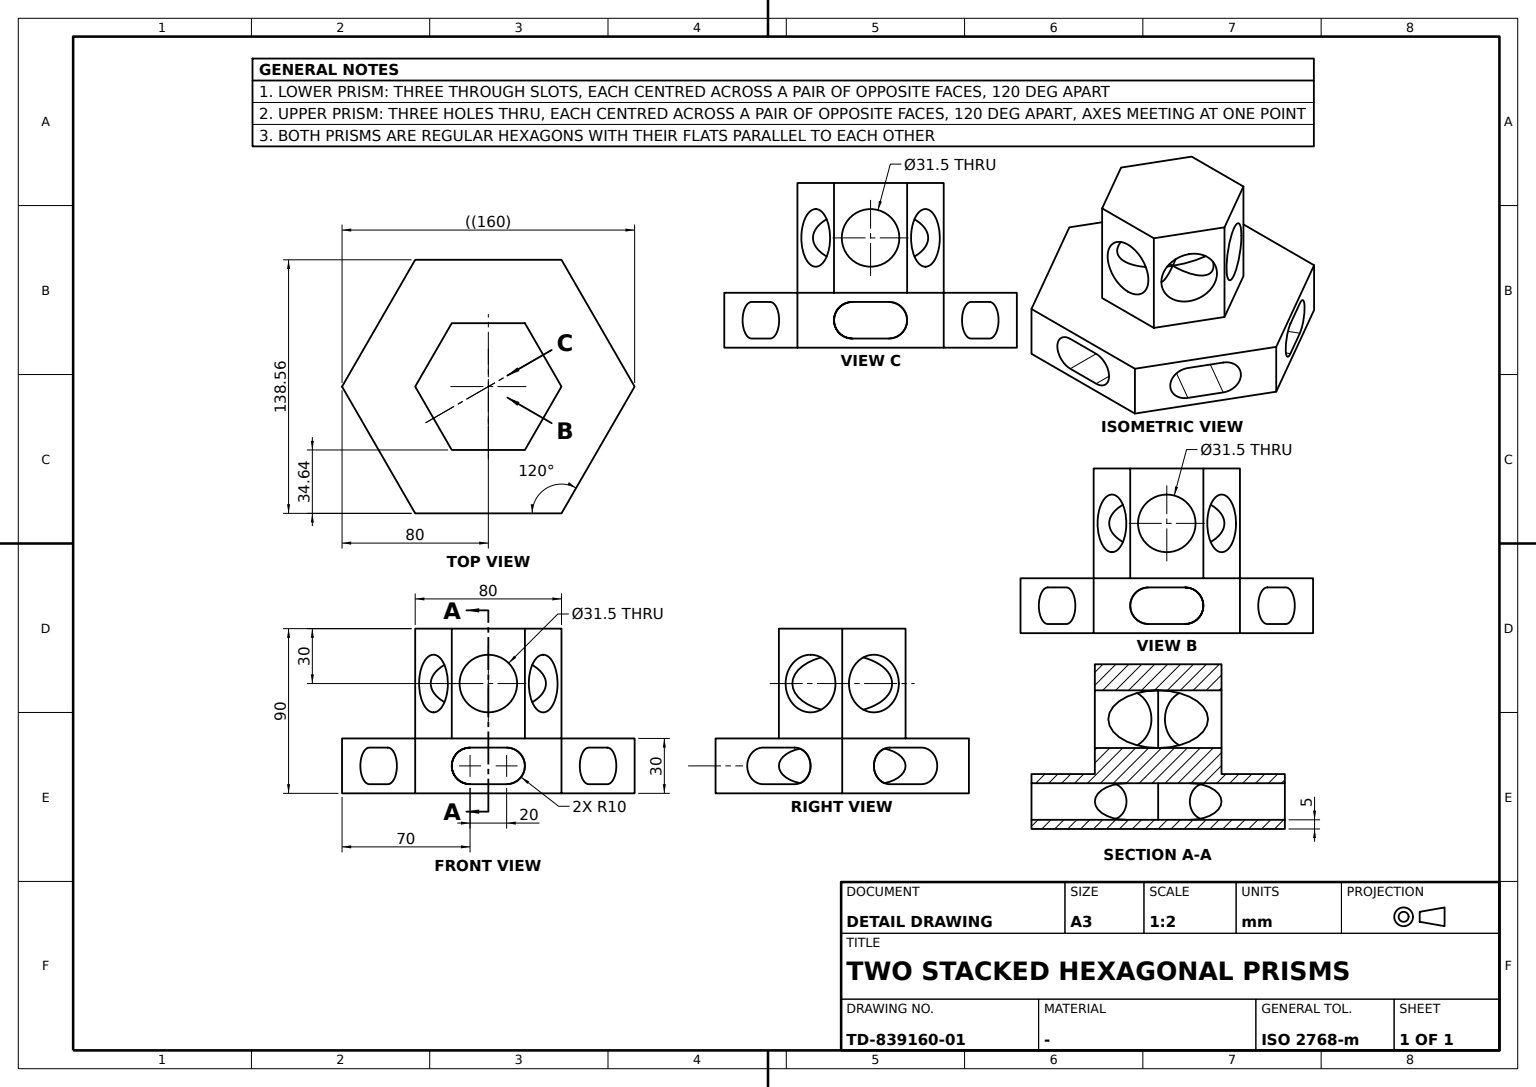
ISO-10303-21;
HEADER;
FILE_DESCRIPTION((''),'2;1');
FILE_NAME('','',(''),(''),'','','');
FILE_SCHEMA(('AUTOMOTIVE_DESIGN'));
ENDSEC;
DATA;
#1=APPLICATION_CONTEXT('');
#2=PRODUCT_CONTEXT('',#1,'mechanical');
#3=PRODUCT('','','',(#2));
#4=PRODUCT_DEFINITION_FORMATION('','',#3);
#5=PRODUCT_DEFINITION_CONTEXT('',#1,'design');
#6=PRODUCT_DEFINITION('','',#4,#5);
#7=PRODUCT_DEFINITION_SHAPE('','',#6);
#8=(LENGTH_UNIT()NAMED_UNIT(*)SI_UNIT(.MILLI.,.METRE.));
#9=(NAMED_UNIT(*)PLANE_ANGLE_UNIT()SI_UNIT($,.RADIAN.));
#10=(NAMED_UNIT(*)SI_UNIT($,.STERADIAN.)SOLID_ANGLE_UNIT());
#11=UNCERTAINTY_MEASURE_WITH_UNIT(LENGTH_MEASURE(0.005),#8,'distance_accuracy_value','');
#12=(GEOMETRIC_REPRESENTATION_CONTEXT(3)GLOBAL_UNCERTAINTY_ASSIGNED_CONTEXT((#11))GLOBAL_UNIT_ASSIGNED_CONTEXT((#8,#9,#10))REPRESENTATION_CONTEXT('',''));
#13=CARTESIAN_POINT('',(-20.,0.,5.));
#14=VERTEX_POINT('',#13);
#15=CARTESIAN_POINT('',(-65.,-25.980762,5.));
#16=VERTEX_POINT('',#15);
#17=CARTESIAN_POINT('',(-35.622295,-9.019536,5.));
#18=DIRECTION('',(0.866025404,0.5,0.));
#19=VECTOR('',#18,1000.);
#20=LINE('',#17,#19);
#21=EDGE_CURVE('',#14,#16,#20,.F.);
#22=ORIENTED_EDGE('',*,*,#21,.F.);
#23=CARTESIAN_POINT('',(-20.,0.,25.));
#24=VERTEX_POINT('',#23);
#25=CARTESIAN_POINT('',(-20.,0.,15.));
#26=DIRECTION('',(0.,1.,0.));
#27=DIRECTION('',(1.,0.,0.));
#28=AXIS2_PLACEMENT_3D('',#25,#26,#27);
#29=ELLIPSE('',#28,20.,10.);
#30=EDGE_CURVE('',#14,#24,#29,.T.);
#31=ORIENTED_EDGE('',*,*,#30,.T.);
#32=CARTESIAN_POINT('',(-65.,-25.980762,25.));
#33=VERTEX_POINT('',#32);
#34=CARTESIAN_POINT('',(-35.622295,-9.019536,25.));
#35=LINE('',#34,#19);
#36=EDGE_CURVE('',#24,#33,#35,.F.);
#37=ORIENTED_EDGE('',*,*,#36,.T.);
#38=CARTESIAN_POINT('',(-65.,-25.980762,15.));
#39=DIRECTION('',(-0.866025404,-0.5,0.));
#40=DIRECTION('',(0.5,-0.866025404,0.));
#41=AXIS2_PLACEMENT_3D('',#38,#39,#40);
#42=CIRCLE('',#41,10.);
#43=EDGE_CURVE('',#33,#16,#42,.T.);
#44=ORIENTED_EDGE('',*,*,#43,.T.);
#45=EDGE_LOOP('',(#22,#31,#37,#44));
#46=FACE_BOUND('',#45,.T.);
#47=CARTESIAN_POINT('',(-35.622295,-9.019536,15.));
#48=DIRECTION('',(-0.5,0.866025404,0.));
#49=AXIS2_PLACEMENT_3D('',#47,#18,#48);
#50=CYLINDRICAL_SURFACE('',#49,10.);
#51=ADVANCED_FACE('',(#46),#50,.F.);
#52=CARTESIAN_POINT('',(-20.,34.641016,30.));
#53=VERTEX_POINT('',#52);
#54=CARTESIAN_POINT('',(-40.,0.,30.));
#55=VERTEX_POINT('',#54);
#56=CARTESIAN_POINT('',(-30.,17.320508,30.));
#57=DIRECTION('',(-0.5,-0.866025404,0.));
#58=VECTOR('',#57,1000.);
#59=LINE('',#56,#58);
#60=EDGE_CURVE('',#53,#55,#59,.T.);
#61=ORIENTED_EDGE('',*,*,#60,.F.);
#62=CARTESIAN_POINT('',(20.,34.641016,30.));
#63=VERTEX_POINT('',#62);
#64=CARTESIAN_POINT('',(0.,34.641016,30.));
#65=DIRECTION('',(-1.,0.,0.));
#66=VECTOR('',#65,1000.);
#67=LINE('',#64,#66);
#68=EDGE_CURVE('',#63,#53,#67,.T.);
#69=ORIENTED_EDGE('',*,*,#68,.F.);
#70=CARTESIAN_POINT('',(40.,0.,30.));
#71=VERTEX_POINT('',#70);
#72=CARTESIAN_POINT('',(30.,17.320508,30.));
#73=VECTOR('',#48,1000.);
#74=LINE('',#72,#73);
#75=EDGE_CURVE('',#71,#63,#74,.T.);
#76=ORIENTED_EDGE('',*,*,#75,.F.);
#77=CARTESIAN_POINT('',(20.,-34.641016,30.));
#78=VERTEX_POINT('',#77);
#79=CARTESIAN_POINT('',(30.,-17.320508,30.));
#80=DIRECTION('',(0.5,0.866025404,0.));
#81=VECTOR('',#80,1000.);
#82=LINE('',#79,#81);
#83=EDGE_CURVE('',#78,#71,#82,.T.);
#84=ORIENTED_EDGE('',*,*,#83,.F.);
#85=CARTESIAN_POINT('',(-20.,-34.641016,30.));
#86=VERTEX_POINT('',#85);
#87=CARTESIAN_POINT('',(0.,-34.641016,30.));
#88=VECTOR('',#27,1000.);
#89=LINE('',#87,#88);
#90=EDGE_CURVE('',#86,#78,#89,.T.);
#91=ORIENTED_EDGE('',*,*,#90,.F.);
#92=CARTESIAN_POINT('',(-30.,-17.320508,30.));
#93=VECTOR('',#40,1000.);
#94=LINE('',#92,#93);
#95=EDGE_CURVE('',#55,#86,#94,.T.);
#96=ORIENTED_EDGE('',*,*,#95,.F.);
#97=EDGE_LOOP('',(#61,#69,#76,#84,#91,#96));
#98=FACE_BOUND('',#97,.T.);
#99=CARTESIAN_POINT('',(40.,-69.282032,30.));
#100=VERTEX_POINT('',#99);
#101=CARTESIAN_POINT('',(80.,0.,30.));
#102=VERTEX_POINT('',#101);
#103=CARTESIAN_POINT('',(60.,-34.641016,30.));
#104=LINE('',#103,#81);
#105=EDGE_CURVE('',#100,#102,#104,.T.);
#106=ORIENTED_EDGE('',*,*,#105,.T.);
#107=CARTESIAN_POINT('',(40.,69.282032,30.));
#108=VERTEX_POINT('',#107);
#109=CARTESIAN_POINT('',(60.,34.641016,30.));
#110=LINE('',#109,#73);
#111=EDGE_CURVE('',#102,#108,#110,.T.);
#112=ORIENTED_EDGE('',*,*,#111,.T.);
#113=CARTESIAN_POINT('',(-40.,69.282032,30.));
#114=VERTEX_POINT('',#113);
#115=CARTESIAN_POINT('',(0.,69.282032,30.));
#116=LINE('',#115,#66);
#117=EDGE_CURVE('',#108,#114,#116,.T.);
#118=ORIENTED_EDGE('',*,*,#117,.T.);
#119=CARTESIAN_POINT('',(-80.,0.,30.));
#120=VERTEX_POINT('',#119);
#121=CARTESIAN_POINT('',(-60.,34.641016,30.));
#122=LINE('',#121,#58);
#123=EDGE_CURVE('',#114,#120,#122,.T.);
#124=ORIENTED_EDGE('',*,*,#123,.T.);
#125=CARTESIAN_POINT('',(-40.,-69.282032,30.));
#126=VERTEX_POINT('',#125);
#127=CARTESIAN_POINT('',(-60.,-34.641016,30.));
#128=LINE('',#127,#93);
#129=EDGE_CURVE('',#120,#126,#128,.T.);
#130=ORIENTED_EDGE('',*,*,#129,.T.);
#131=CARTESIAN_POINT('',(0.,-69.282032,30.));
#132=LINE('',#131,#88);
#133=EDGE_CURVE('',#126,#100,#132,.T.);
#134=ORIENTED_EDGE('',*,*,#133,.T.);
#135=EDGE_LOOP('',(#106,#112,#118,#124,#130,#134));
#136=FACE_BOUND('',#135,.T.);
#137=CARTESIAN_POINT('',(0.,0.,30.));
#138=DIRECTION('',(0.,0.,1.));
#139=AXIS2_PLACEMENT_3D('',#137,#138,#27);
#140=PLANE('',#139);
#141=ADVANCED_FACE('',(#98,#136),#140,.T.);
#142=CARTESIAN_POINT('',(-40.,0.,90.));
#143=VERTEX_POINT('',#142);
#144=CARTESIAN_POINT('',(-20.,-34.641016,90.));
#145=VERTEX_POINT('',#144);
#146=CARTESIAN_POINT('',(-30.,-17.320508,90.));
#147=LINE('',#146,#93);
#148=EDGE_CURVE('',#143,#145,#147,.T.);
#149=ORIENTED_EDGE('',*,*,#148,.T.);
#150=CARTESIAN_POINT('',(20.,-34.641016,90.));
#151=VERTEX_POINT('',#150);
#152=CARTESIAN_POINT('',(0.,-34.641016,90.));
#153=LINE('',#152,#88);
#154=EDGE_CURVE('',#145,#151,#153,.T.);
#155=ORIENTED_EDGE('',*,*,#154,.T.);
#156=CARTESIAN_POINT('',(40.,0.,90.));
#157=VERTEX_POINT('',#156);
#158=CARTESIAN_POINT('',(30.,-17.320508,90.));
#159=LINE('',#158,#81);
#160=EDGE_CURVE('',#151,#157,#159,.T.);
#161=ORIENTED_EDGE('',*,*,#160,.T.);
#162=CARTESIAN_POINT('',(20.,34.641016,90.));
#163=VERTEX_POINT('',#162);
#164=CARTESIAN_POINT('',(30.,17.320508,90.));
#165=LINE('',#164,#73);
#166=EDGE_CURVE('',#157,#163,#165,.T.);
#167=ORIENTED_EDGE('',*,*,#166,.T.);
#168=CARTESIAN_POINT('',(-20.,34.641016,90.));
#169=VERTEX_POINT('',#168);
#170=CARTESIAN_POINT('',(0.,34.641016,90.));
#171=LINE('',#170,#66);
#172=EDGE_CURVE('',#163,#169,#171,.T.);
#173=ORIENTED_EDGE('',*,*,#172,.T.);
#174=CARTESIAN_POINT('',(-30.,17.320508,90.));
#175=LINE('',#174,#58);
#176=EDGE_CURVE('',#169,#143,#175,.T.);
#177=ORIENTED_EDGE('',*,*,#176,.T.);
#178=EDGE_LOOP('',(#149,#155,#161,#167,#173,#177));
#179=FACE_BOUND('',#178,.T.);
#180=CARTESIAN_POINT('',(0.,0.,90.));
#181=AXIS2_PLACEMENT_3D('',#180,#138,#27);
#182=PLANE('',#181);
#183=ADVANCED_FACE('',(#179),#182,.T.);
#184=ORIENTED_EDGE('',*,*,#117,.F.);
#185=CARTESIAN_POINT('',(40.,69.282032,0.));
#186=VERTEX_POINT('',#185);
#187=VECTOR('',#138,1000.);
#188=LINE('',#185,#187);
#189=EDGE_CURVE('',#186,#108,#188,.T.);
#190=ORIENTED_EDGE('',*,*,#189,.F.);
#191=CARTESIAN_POINT('',(-40.,69.282032,0.));
#192=VERTEX_POINT('',#191);
#193=CARTESIAN_POINT('',(0.,69.282032,0.));
#194=LINE('',#193,#66);
#195=EDGE_CURVE('',#186,#192,#194,.T.);
#196=ORIENTED_EDGE('',*,*,#195,.T.);
#197=LINE('',#191,#187);
#198=EDGE_CURVE('',#192,#114,#197,.T.);
#199=ORIENTED_EDGE('',*,*,#198,.T.);
#200=EDGE_LOOP('',(#184,#190,#196,#199));
#201=FACE_BOUND('',#200,.T.);
#202=CARTESIAN_POINT('',(10.,69.282032,5.));
#203=VERTEX_POINT('',#202);
#204=CARTESIAN_POINT('',(-10.,69.282032,5.));
#205=VERTEX_POINT('',#204);
#206=CARTESIAN_POINT('',(40.,69.282032,5.));
#207=LINE('',#206,#66);
#208=EDGE_CURVE('',#203,#205,#207,.T.);
#209=ORIENTED_EDGE('',*,*,#208,.F.);
#210=CARTESIAN_POINT('',(10.,69.282032,25.));
#211=VERTEX_POINT('',#210);
#212=CARTESIAN_POINT('',(10.,69.282032,15.));
#213=AXIS2_PLACEMENT_3D('',#212,#26,#65);
#214=CIRCLE('',#213,10.);
#215=EDGE_CURVE('',#211,#203,#214,.T.);
#216=ORIENTED_EDGE('',*,*,#215,.F.);
#217=CARTESIAN_POINT('',(-10.,69.282032,25.));
#218=VERTEX_POINT('',#217);
#219=CARTESIAN_POINT('',(40.,69.282032,25.));
#220=LINE('',#219,#88);
#221=EDGE_CURVE('',#218,#211,#220,.T.);
#222=ORIENTED_EDGE('',*,*,#221,.F.);
#223=CARTESIAN_POINT('',(-10.,69.282032,15.));
#224=AXIS2_PLACEMENT_3D('',#223,#26,#65);
#225=CIRCLE('',#224,10.);
#226=EDGE_CURVE('',#205,#218,#225,.T.);
#227=ORIENTED_EDGE('',*,*,#226,.F.);
#228=EDGE_LOOP('',(#209,#216,#222,#227));
#229=FACE_BOUND('',#228,.T.);
#230=AXIS2_PLACEMENT_3D('',#185,#26,#65);
#231=PLANE('',#230);
#232=ADVANCED_FACE('',(#201,#229),#231,.T.);
#233=CARTESIAN_POINT('',(0.,0.,44.25));
#234=VERTEX_POINT('',#233);
#235=CARTESIAN_POINT('',(0.,0.,75.75));
#236=VERTEX_POINT('',#235);
#237=CARTESIAN_POINT('',(0.,0.,60.));
#238=DIRECTION('',(0.866025404,-0.5,0.));
#239=AXIS2_PLACEMENT_3D('',#237,#238,#57);
#240=ELLIPSE('',#239,31.5,15.75);
#241=EDGE_CURVE('',#234,#236,#240,.T.);
#242=ORIENTED_EDGE('',*,*,#241,.F.);
#243=AXIS2_PLACEMENT_3D('',#237,#26,#65);
#244=ELLIPSE('',#243,31.5,15.75);
#245=EDGE_CURVE('',#236,#234,#244,.T.);
#246=ORIENTED_EDGE('',*,*,#245,.F.);
#247=EDGE_LOOP('',(#242,#246));
#248=FACE_BOUND('',#247,.T.);
#249=CARTESIAN_POINT('',(22.125,30.960408,60.));
#250=VERTEX_POINT('',#249);
#251=CARTESIAN_POINT('',(30.,17.320508,60.));
#252=AXIS2_PLACEMENT_3D('',#251,#18,#48);
#253=CIRCLE('',#252,15.75);
#254=EDGE_CURVE('',#250,#250,#253,.T.);
#255=ORIENTED_EDGE('',*,*,#254,.T.);
#256=EDGE_LOOP('',(#255));
#257=FACE_BOUND('',#256,.T.);
#258=CARTESIAN_POINT('',(-51.809795,-29.912399,60.));
#259=AXIS2_PLACEMENT_3D('',#258,#18,#48);
#260=CYLINDRICAL_SURFACE('',#259,15.75);
#261=ADVANCED_FACE('',(#248,#257),#260,.F.);
#262=CARTESIAN_POINT('',(80.,0.,0.));
#263=VERTEX_POINT('',#262);
#264=LINE('',#262,#187);
#265=EDGE_CURVE('',#263,#102,#264,.T.);
#266=ORIENTED_EDGE('',*,*,#265,.F.);
#267=CARTESIAN_POINT('',(60.,34.641016,0.));
#268=LINE('',#267,#73);
#269=EDGE_CURVE('',#263,#186,#268,.T.);
#270=ORIENTED_EDGE('',*,*,#269,.T.);
#271=ORIENTED_EDGE('',*,*,#189,.T.);
#272=ORIENTED_EDGE('',*,*,#111,.F.);
#273=EDGE_LOOP('',(#266,#270,#271,#272));
#274=FACE_BOUND('',#273,.T.);
#275=CARTESIAN_POINT('',(65.,25.980762,25.));
#276=VERTEX_POINT('',#275);
#277=CARTESIAN_POINT('',(65.,25.980762,5.));
#278=VERTEX_POINT('',#277);
#279=CARTESIAN_POINT('',(65.,25.980762,15.));
#280=AXIS2_PLACEMENT_3D('',#279,#18,#48);
#281=CIRCLE('',#280,10.);
#282=EDGE_CURVE('',#276,#278,#281,.T.);
#283=ORIENTED_EDGE('',*,*,#282,.F.);
#284=CARTESIAN_POINT('',(55.,43.30127,25.));
#285=VERTEX_POINT('',#284);
#286=LINE('',#275,#73);
#287=EDGE_CURVE('',#276,#285,#286,.T.);
#288=ORIENTED_EDGE('',*,*,#287,.T.);
#289=CARTESIAN_POINT('',(55.,43.30127,5.));
#290=VERTEX_POINT('',#289);
#291=CARTESIAN_POINT('',(55.,43.30127,15.));
#292=AXIS2_PLACEMENT_3D('',#291,#18,#48);
#293=CIRCLE('',#292,10.);
#294=EDGE_CURVE('',#290,#285,#293,.T.);
#295=ORIENTED_EDGE('',*,*,#294,.F.);
#296=LINE('',#289,#93);
#297=EDGE_CURVE('',#290,#278,#296,.T.);
#298=ORIENTED_EDGE('',*,*,#297,.T.);
#299=EDGE_LOOP('',(#283,#288,#295,#298));
#300=FACE_BOUND('',#299,.T.);
#301=AXIS2_PLACEMENT_3D('',#262,#18,#48);
#302=PLANE('',#301);
#303=ADVANCED_FACE('',(#274,#300),#302,.T.);
#304=ORIENTED_EDGE('',*,*,#198,.F.);
#305=CARTESIAN_POINT('',(-80.,0.,0.));
#306=VERTEX_POINT('',#305);
#307=CARTESIAN_POINT('',(-60.,34.641016,0.));
#308=LINE('',#307,#58);
#309=EDGE_CURVE('',#192,#306,#308,.T.);
#310=ORIENTED_EDGE('',*,*,#309,.T.);
#311=LINE('',#305,#187);
#312=EDGE_CURVE('',#306,#120,#311,.T.);
#313=ORIENTED_EDGE('',*,*,#312,.T.);
#314=ORIENTED_EDGE('',*,*,#123,.F.);
#315=EDGE_LOOP('',(#304,#310,#313,#314));
#316=FACE_BOUND('',#315,.T.);
#317=CARTESIAN_POINT('',(-55.,43.30127,25.));
#318=VERTEX_POINT('',#317);
#319=CARTESIAN_POINT('',(-65.,25.980762,25.));
#320=VERTEX_POINT('',#319);
#321=CARTESIAN_POINT('',(-32.5,82.272413,25.));
#322=LINE('',#321,#58);
#323=EDGE_CURVE('',#318,#320,#322,.T.);
#324=ORIENTED_EDGE('',*,*,#323,.T.);
#325=CARTESIAN_POINT('',(-65.,25.980762,5.));
#326=VERTEX_POINT('',#325);
#327=CARTESIAN_POINT('',(-65.,25.980762,15.));
#328=DIRECTION('',(-0.866025404,0.5,0.));
#329=AXIS2_PLACEMENT_3D('',#327,#328,#57);
#330=CIRCLE('',#329,10.);
#331=EDGE_CURVE('',#326,#320,#330,.T.);
#332=ORIENTED_EDGE('',*,*,#331,.F.);
#333=CARTESIAN_POINT('',(-55.,43.30127,5.));
#334=VERTEX_POINT('',#333);
#335=CARTESIAN_POINT('',(-27.5,90.932667,5.));
#336=LINE('',#335,#81);
#337=EDGE_CURVE('',#326,#334,#336,.T.);
#338=ORIENTED_EDGE('',*,*,#337,.T.);
#339=CARTESIAN_POINT('',(-55.,43.30127,15.));
#340=AXIS2_PLACEMENT_3D('',#339,#328,#57);
#341=CIRCLE('',#340,10.);
#342=EDGE_CURVE('',#318,#334,#341,.T.);
#343=ORIENTED_EDGE('',*,*,#342,.F.);
#344=EDGE_LOOP('',(#324,#332,#338,#343));
#345=FACE_BOUND('',#344,.T.);
#346=AXIS2_PLACEMENT_3D('',#191,#328,#57);
#347=PLANE('',#346);
#348=ADVANCED_FACE('',(#316,#345),#347,.T.);
#349=CARTESIAN_POINT('',(10.,-69.282032,5.));
#350=VERTEX_POINT('',#349);
#351=CARTESIAN_POINT('',(10.,-17.320508,5.));
#352=VERTEX_POINT('',#351);
#353=CARTESIAN_POINT('',(10.,35.35958,5.));
#354=DIRECTION('',(0.,-1.,0.));
#355=VECTOR('',#354,1000.);
#356=LINE('',#353,#355);
#357=EDGE_CURVE('',#350,#352,#356,.F.);
#358=ORIENTED_EDGE('',*,*,#357,.F.);
#359=CARTESIAN_POINT('',(10.,-69.282032,25.));
#360=VERTEX_POINT('',#359);
#361=CARTESIAN_POINT('',(10.,-69.282032,15.));
#362=DIRECTION('',(0.,0.,-1.));
#363=AXIS2_PLACEMENT_3D('',#361,#354,#362);
#364=CIRCLE('',#363,10.);
#365=EDGE_CURVE('',#350,#360,#364,.T.);
#366=ORIENTED_EDGE('',*,*,#365,.T.);
#367=CARTESIAN_POINT('',(10.,-17.320508,25.));
#368=VERTEX_POINT('',#367);
#369=CARTESIAN_POINT('',(10.,35.35958,25.));
#370=LINE('',#369,#355);
#371=EDGE_CURVE('',#360,#368,#370,.F.);
#372=ORIENTED_EDGE('',*,*,#371,.T.);
#373=CARTESIAN_POINT('',(10.,-17.320508,15.));
#374=AXIS2_PLACEMENT_3D('',#373,#39,#48);
#375=ELLIPSE('',#374,20.,10.);
#376=EDGE_CURVE('',#352,#368,#375,.T.);
#377=ORIENTED_EDGE('',*,*,#376,.F.);
#378=EDGE_LOOP('',(#358,#366,#372,#377));
#379=FACE_BOUND('',#378,.T.);
#380=CARTESIAN_POINT('',(10.,35.35958,15.));
#381=AXIS2_PLACEMENT_3D('',#380,#354,#27);
#382=CYLINDRICAL_SURFACE('',#381,10.);
#383=ADVANCED_FACE('',(#379),#382,.F.);
#384=CARTESIAN_POINT('',(-10.,-69.282032,25.));
#385=VERTEX_POINT('',#384);
#386=CARTESIAN_POINT('',(65.,-69.282032,25.));
#387=LINE('',#386,#88);
#388=EDGE_CURVE('',#385,#360,#387,.T.);
#389=ORIENTED_EDGE('',*,*,#388,.F.);
#390=CARTESIAN_POINT('',(-10.,-17.320508,25.));
#391=VERTEX_POINT('',#390);
#392=CARTESIAN_POINT('',(-10.,35.35958,25.));
#393=LINE('',#392,#355);
#394=EDGE_CURVE('',#385,#391,#393,.F.);
#395=ORIENTED_EDGE('',*,*,#394,.T.);
#396=CARTESIAN_POINT('',(-55.,-43.30127,25.));
#397=VERTEX_POINT('',#396);
#398=CARTESIAN_POINT('',(-25.622295,-26.340044,25.));
#399=LINE('',#398,#19);
#400=EDGE_CURVE('',#391,#397,#399,.F.);
#401=ORIENTED_EDGE('',*,*,#400,.T.);
#402=CARTESIAN_POINT('',(-80.,0.,25.));
#403=LINE('',#402,#73);
#404=EDGE_CURVE('',#397,#33,#403,.T.);
#405=ORIENTED_EDGE('',*,*,#404,.T.);
#406=ORIENTED_EDGE('',*,*,#36,.F.);
#407=CARTESIAN_POINT('',(25.622295,-26.340044,25.));
#408=VECTOR('',#328,1000.);
#409=LINE('',#407,#408);
#410=EDGE_CURVE('',#320,#24,#409,.F.);
#411=ORIENTED_EDGE('',*,*,#410,.F.);
#412=ORIENTED_EDGE('',*,*,#323,.F.);
#413=CARTESIAN_POINT('',(-10.,17.320508,25.));
#414=VERTEX_POINT('',#413);
#415=CARTESIAN_POINT('',(35.622295,-9.019536,25.));
#416=LINE('',#415,#408);
#417=EDGE_CURVE('',#318,#414,#416,.F.);
#418=ORIENTED_EDGE('',*,*,#417,.T.);
#419=EDGE_CURVE('',#414,#218,#393,.F.);
#420=ORIENTED_EDGE('',*,*,#419,.T.);
#421=ORIENTED_EDGE('',*,*,#221,.T.);
#422=CARTESIAN_POINT('',(10.,17.320508,25.));
#423=VERTEX_POINT('',#422);
#424=EDGE_CURVE('',#423,#211,#370,.F.);
#425=ORIENTED_EDGE('',*,*,#424,.F.);
#426=EDGE_CURVE('',#285,#423,#35,.F.);
#427=ORIENTED_EDGE('',*,*,#426,.F.);
#428=ORIENTED_EDGE('',*,*,#287,.F.);
#429=CARTESIAN_POINT('',(20.,0.,25.));
#430=VERTEX_POINT('',#429);
#431=EDGE_CURVE('',#276,#430,#399,.F.);
#432=ORIENTED_EDGE('',*,*,#431,.T.);
#433=CARTESIAN_POINT('',(65.,-25.980762,25.));
#434=VERTEX_POINT('',#433);
#435=EDGE_CURVE('',#430,#434,#416,.F.);
#436=ORIENTED_EDGE('',*,*,#435,.T.);
#437=CARTESIAN_POINT('',(55.,-43.30127,25.));
#438=VERTEX_POINT('',#437);
#439=CARTESIAN_POINT('',(40.,-69.282032,25.));
#440=LINE('',#439,#58);
#441=EDGE_CURVE('',#434,#438,#440,.T.);
#442=ORIENTED_EDGE('',*,*,#441,.T.);
#443=EDGE_CURVE('',#368,#438,#409,.F.);
#444=ORIENTED_EDGE('',*,*,#443,.F.);
#445=ORIENTED_EDGE('',*,*,#371,.F.);
#446=EDGE_LOOP('',(#389,#395,#401,#405,#406,#411,#412,#418,#420,#421,#425,#427,#428,#432,#436,#442,#444,#445));
#447=FACE_BOUND('',#446,.T.);
#448=AXIS2_PLACEMENT_3D('',#275,#138,#48);
#449=PLANE('',#448);
#450=ADVANCED_FACE('',(#447),#449,.F.);
#451=CARTESIAN_POINT('',(37.875,-3.680608,60.));
#452=VERTEX_POINT('',#451);
#453=CARTESIAN_POINT('',(30.,-17.320508,60.));
#454=AXIS2_PLACEMENT_3D('',#453,#238,#80);
#455=CIRCLE('',#454,15.75);
#456=EDGE_CURVE('',#452,#452,#455,.T.);
#457=ORIENTED_EDGE('',*,*,#456,.T.);
#458=EDGE_LOOP('',(#457));
#459=FACE_BOUND('',#458,.T.);
#460=AXIS2_PLACEMENT_3D('',#237,#39,#40);
#461=ELLIPSE('',#460,31.5,15.75);
#462=EDGE_CURVE('',#236,#234,#461,.F.);
#463=ORIENTED_EDGE('',*,*,#462,.F.);
#464=ORIENTED_EDGE('',*,*,#245,.T.);
#465=EDGE_LOOP('',(#463,#464));
#466=FACE_BOUND('',#465,.T.);
#467=CARTESIAN_POINT('',(51.809795,-29.912399,60.));
#468=AXIS2_PLACEMENT_3D('',#467,#328,#57);
#469=CYLINDRICAL_SURFACE('',#468,15.75);
#470=ADVANCED_FACE('',(#459,#466),#469,.F.);
#471=ORIENTED_EDGE('',*,*,#435,.F.);
#472=CARTESIAN_POINT('',(20.,0.,5.));
#473=VERTEX_POINT('',#472);
#474=CARTESIAN_POINT('',(20.,0.,15.));
#475=AXIS2_PLACEMENT_3D('',#474,#26,#27);
#476=ELLIPSE('',#475,20.,10.);
#477=EDGE_CURVE('',#473,#430,#476,.F.);
#478=ORIENTED_EDGE('',*,*,#477,.F.);
#479=CARTESIAN_POINT('',(65.,-25.980762,5.));
#480=VERTEX_POINT('',#479);
#481=CARTESIAN_POINT('',(35.622295,-9.019536,5.));
#482=LINE('',#481,#408);
#483=EDGE_CURVE('',#473,#480,#482,.F.);
#484=ORIENTED_EDGE('',*,*,#483,.T.);
#485=CARTESIAN_POINT('',(65.,-25.980762,15.));
#486=AXIS2_PLACEMENT_3D('',#485,#238,#80);
#487=CIRCLE('',#486,10.);
#488=EDGE_CURVE('',#480,#434,#487,.T.);
#489=ORIENTED_EDGE('',*,*,#488,.T.);
#490=EDGE_LOOP('',(#471,#478,#484,#489));
#491=FACE_BOUND('',#490,.T.);
#492=CARTESIAN_POINT('',(35.622295,-9.019536,15.));
#493=AXIS2_PLACEMENT_3D('',#492,#328,#57);
#494=CYLINDRICAL_SURFACE('',#493,10.);
#495=ADVANCED_FACE('',(#491),#494,.F.);
#496=CARTESIAN_POINT('',(-10.,-69.282032,5.));
#497=VERTEX_POINT('',#496);
#498=CARTESIAN_POINT('',(-10.,-17.320508,5.));
#499=VERTEX_POINT('',#498);
#500=CARTESIAN_POINT('',(-10.,35.35958,5.));
#501=LINE('',#500,#355);
#502=EDGE_CURVE('',#497,#499,#501,.F.);
#503=ORIENTED_EDGE('',*,*,#502,.T.);
#504=CARTESIAN_POINT('',(-10.,-17.320508,15.));
#505=AXIS2_PLACEMENT_3D('',#504,#238,#80);
#506=ELLIPSE('',#505,20.,10.);
#507=EDGE_CURVE('',#391,#499,#506,.T.);
#508=ORIENTED_EDGE('',*,*,#507,.F.);
#509=ORIENTED_EDGE('',*,*,#394,.F.);
#510=CARTESIAN_POINT('',(-10.,-69.282032,15.));
#511=AXIS2_PLACEMENT_3D('',#510,#354,#362);
#512=CIRCLE('',#511,10.);
#513=EDGE_CURVE('',#385,#497,#512,.T.);
#514=ORIENTED_EDGE('',*,*,#513,.T.);
#515=EDGE_LOOP('',(#503,#508,#509,#514));
#516=FACE_BOUND('',#515,.T.);
#517=CARTESIAN_POINT('',(-10.,35.35958,15.));
#518=AXIS2_PLACEMENT_3D('',#517,#354,#27);
#519=CYLINDRICAL_SURFACE('',#518,10.);
#520=ADVANCED_FACE('',(#516),#519,.F.);
#521=CARTESIAN_POINT('',(-10.,17.320508,5.));
#522=VERTEX_POINT('',#521);
#523=CARTESIAN_POINT('',(-10.,17.320508,15.));
#524=AXIS2_PLACEMENT_3D('',#523,#39,#48);
#525=ELLIPSE('',#524,20.,10.);
#526=EDGE_CURVE('',#522,#414,#525,.F.);
#527=ORIENTED_EDGE('',*,*,#526,.F.);
#528=EDGE_CURVE('',#522,#205,#501,.F.);
#529=ORIENTED_EDGE('',*,*,#528,.T.);
#530=ORIENTED_EDGE('',*,*,#226,.T.);
#531=ORIENTED_EDGE('',*,*,#419,.F.);
#532=EDGE_LOOP('',(#527,#529,#530,#531));
#533=FACE_BOUND('',#532,.T.);
#534=ADVANCED_FACE('',(#533),#519,.F.);
#535=CARTESIAN_POINT('',(40.,-69.282032,0.));
#536=VERTEX_POINT('',#535);
#537=CARTESIAN_POINT('',(60.,-34.641016,0.));
#538=LINE('',#537,#81);
#539=EDGE_CURVE('',#536,#263,#538,.T.);
#540=ORIENTED_EDGE('',*,*,#539,.F.);
#541=CARTESIAN_POINT('',(-40.,-69.282032,0.));
#542=VERTEX_POINT('',#541);
#543=CARTESIAN_POINT('',(0.,-69.282032,0.));
#544=LINE('',#543,#88);
#545=EDGE_CURVE('',#542,#536,#544,.T.);
#546=ORIENTED_EDGE('',*,*,#545,.F.);
#547=CARTESIAN_POINT('',(-60.,-34.641016,0.));
#548=LINE('',#547,#93);
#549=EDGE_CURVE('',#306,#542,#548,.T.);
#550=ORIENTED_EDGE('',*,*,#549,.F.);
#551=ORIENTED_EDGE('',*,*,#309,.F.);
#552=ORIENTED_EDGE('',*,*,#195,.F.);
#553=ORIENTED_EDGE('',*,*,#269,.F.);
#554=EDGE_LOOP('',(#540,#546,#550,#551,#552,#553));
#555=FACE_BOUND('',#554,.T.);
#556=CARTESIAN_POINT('',(0.,0.,0.));
#557=AXIS2_PLACEMENT_3D('',#556,#138,#27);
#558=PLANE('',#557);
#559=ADVANCED_FACE('',(#555),#558,.F.);
#560=ORIENTED_EDGE('',*,*,#105,.F.);
#561=LINE('',#535,#187);
#562=EDGE_CURVE('',#536,#100,#561,.T.);
#563=ORIENTED_EDGE('',*,*,#562,.F.);
#564=ORIENTED_EDGE('',*,*,#539,.T.);
#565=ORIENTED_EDGE('',*,*,#265,.T.);
#566=EDGE_LOOP('',(#560,#563,#564,#565));
#567=FACE_BOUND('',#566,.T.);
#568=ORIENTED_EDGE('',*,*,#441,.F.);
#569=ORIENTED_EDGE('',*,*,#488,.F.);
#570=CARTESIAN_POINT('',(55.,-43.30127,5.));
#571=VERTEX_POINT('',#570);
#572=CARTESIAN_POINT('',(40.,-69.282032,5.));
#573=LINE('',#572,#81);
#574=EDGE_CURVE('',#571,#480,#573,.T.);
#575=ORIENTED_EDGE('',*,*,#574,.F.);
#576=CARTESIAN_POINT('',(55.,-43.30127,15.));
#577=AXIS2_PLACEMENT_3D('',#576,#238,#80);
#578=CIRCLE('',#577,10.);
#579=EDGE_CURVE('',#438,#571,#578,.T.);
#580=ORIENTED_EDGE('',*,*,#579,.F.);
#581=EDGE_LOOP('',(#568,#569,#575,#580));
#582=FACE_BOUND('',#581,.T.);
#583=AXIS2_PLACEMENT_3D('',#535,#238,#80);
#584=PLANE('',#583);
#585=ADVANCED_FACE('',(#567,#582),#584,.T.);
#586=ORIENTED_EDGE('',*,*,#513,.F.);
#587=ORIENTED_EDGE('',*,*,#388,.T.);
#588=ORIENTED_EDGE('',*,*,#365,.F.);
#589=CARTESIAN_POINT('',(55.,-69.282032,5.));
#590=LINE('',#589,#66);
#591=EDGE_CURVE('',#350,#497,#590,.T.);
#592=ORIENTED_EDGE('',*,*,#591,.T.);
#593=EDGE_LOOP('',(#586,#587,#588,#592));
#594=FACE_BOUND('',#593,.T.);
#595=ORIENTED_EDGE('',*,*,#133,.F.);
#596=LINE('',#541,#187);
#597=EDGE_CURVE('',#542,#126,#596,.T.);
#598=ORIENTED_EDGE('',*,*,#597,.F.);
#599=ORIENTED_EDGE('',*,*,#545,.T.);
#600=ORIENTED_EDGE('',*,*,#562,.T.);
#601=EDGE_LOOP('',(#595,#598,#599,#600));
#602=FACE_BOUND('',#601,.T.);
#603=AXIS2_PLACEMENT_3D('',#541,#354,#27);
#604=PLANE('',#603);
#605=ADVANCED_FACE('',(#594,#602),#604,.T.);
#606=CARTESIAN_POINT('',(10.,17.320508,5.));
#607=VERTEX_POINT('',#606);
#608=CARTESIAN_POINT('',(10.,17.320508,15.));
#609=AXIS2_PLACEMENT_3D('',#608,#238,#80);
#610=ELLIPSE('',#609,20.,10.);
#611=EDGE_CURVE('',#423,#607,#610,.F.);
#612=ORIENTED_EDGE('',*,*,#611,.F.);
#613=ORIENTED_EDGE('',*,*,#424,.T.);
#614=ORIENTED_EDGE('',*,*,#215,.T.);
#615=EDGE_CURVE('',#607,#203,#356,.F.);
#616=ORIENTED_EDGE('',*,*,#615,.F.);
#617=EDGE_LOOP('',(#612,#613,#614,#616));
#618=FACE_BOUND('',#617,.T.);
#619=ADVANCED_FACE('',(#618),#382,.F.);
#620=ORIENTED_EDGE('',*,*,#95,.T.);
#621=LINE('',#85,#187);
#622=EDGE_CURVE('',#86,#145,#621,.T.);
#623=ORIENTED_EDGE('',*,*,#622,.T.);
#624=ORIENTED_EDGE('',*,*,#148,.F.);
#625=LINE('',#54,#187);
#626=EDGE_CURVE('',#55,#143,#625,.T.);
#627=ORIENTED_EDGE('',*,*,#626,.F.);
#628=EDGE_LOOP('',(#620,#623,#624,#627));
#629=FACE_BOUND('',#628,.T.);
#630=CARTESIAN_POINT('',(-22.125,-30.960408,60.));
#631=VERTEX_POINT('',#630);
#632=CARTESIAN_POINT('',(-30.,-17.320508,60.));
#633=AXIS2_PLACEMENT_3D('',#632,#39,#40);
#634=CIRCLE('',#633,15.75);
#635=EDGE_CURVE('',#631,#631,#634,.T.);
#636=ORIENTED_EDGE('',*,*,#635,.F.);
#637=EDGE_LOOP('',(#636));
#638=FACE_BOUND('',#637,.T.);
#639=AXIS2_PLACEMENT_3D('',#54,#39,#40);
#640=PLANE('',#639);
#641=ADVANCED_FACE('',(#629,#638),#640,.T.);
#642=ORIENTED_EDGE('',*,*,#635,.T.);
#643=EDGE_LOOP('',(#642));
#644=FACE_BOUND('',#643,.T.);
#645=AXIS2_PLACEMENT_3D('',#237,#26,#27);
#646=ELLIPSE('',#645,31.5,15.75);
#647=EDGE_CURVE('',#236,#234,#646,.F.);
#648=ORIENTED_EDGE('',*,*,#647,.F.);
#649=EDGE_CURVE('',#234,#236,#240,.F.);
#650=ORIENTED_EDGE('',*,*,#649,.F.);
#651=EDGE_LOOP('',(#648,#650));
#652=FACE_BOUND('',#651,.T.);
#653=ADVANCED_FACE('',(#644,#652),#260,.F.);
#654=CARTESIAN_POINT('',(25.622295,-26.340044,5.));
#655=LINE('',#654,#408);
#656=EDGE_CURVE('',#326,#14,#655,.F.);
#657=ORIENTED_EDGE('',*,*,#656,.F.);
#658=ORIENTED_EDGE('',*,*,#331,.T.);
#659=ORIENTED_EDGE('',*,*,#410,.T.);
#660=ORIENTED_EDGE('',*,*,#30,.F.);
#661=EDGE_LOOP('',(#657,#658,#659,#660));
#662=FACE_BOUND('',#661,.T.);
#663=CARTESIAN_POINT('',(25.622295,-26.340044,15.));
#664=AXIS2_PLACEMENT_3D('',#663,#328,#57);
#665=CYLINDRICAL_SURFACE('',#664,10.);
#666=ADVANCED_FACE('',(#662),#665,.F.);
#667=CARTESIAN_POINT('',(0.,-34.641016,44.25));
#668=VERTEX_POINT('',#667);
#669=CARTESIAN_POINT('',(0.,-34.641016,60.));
#670=AXIS2_PLACEMENT_3D('',#669,#354,#362);
#671=CIRCLE('',#670,15.75);
#672=EDGE_CURVE('',#668,#668,#671,.T.);
#673=ORIENTED_EDGE('',*,*,#672,.F.);
#674=EDGE_LOOP('',(#673));
#675=FACE_BOUND('',#674,.T.);
#676=LINE('',#77,#187);
#677=EDGE_CURVE('',#78,#151,#676,.T.);
#678=ORIENTED_EDGE('',*,*,#677,.T.);
#679=ORIENTED_EDGE('',*,*,#154,.F.);
#680=ORIENTED_EDGE('',*,*,#622,.F.);
#681=ORIENTED_EDGE('',*,*,#90,.T.);
#682=EDGE_LOOP('',(#678,#679,#680,#681));
#683=FACE_BOUND('',#682,.T.);
#684=AXIS2_PLACEMENT_3D('',#85,#354,#27);
#685=PLANE('',#684);
#686=ADVANCED_FACE('',(#675,#683),#685,.T.);
#687=EDGE_CURVE('',#290,#607,#20,.F.);
#688=ORIENTED_EDGE('',*,*,#687,.F.);
#689=ORIENTED_EDGE('',*,*,#294,.T.);
#690=ORIENTED_EDGE('',*,*,#426,.T.);
#691=ORIENTED_EDGE('',*,*,#611,.T.);
#692=EDGE_LOOP('',(#688,#689,#690,#691));
#693=FACE_BOUND('',#692,.T.);
#694=ADVANCED_FACE('',(#693),#50,.F.);
#695=EDGE_CURVE('',#352,#571,#655,.F.);
#696=ORIENTED_EDGE('',*,*,#695,.F.);
#697=ORIENTED_EDGE('',*,*,#376,.T.);
#698=ORIENTED_EDGE('',*,*,#443,.T.);
#699=ORIENTED_EDGE('',*,*,#579,.T.);
#700=EDGE_LOOP('',(#696,#697,#698,#699));
#701=FACE_BOUND('',#700,.T.);
#702=ADVANCED_FACE('',(#701),#665,.F.);
#703=EDGE_CURVE('',#236,#234,#461,.T.);
#704=ORIENTED_EDGE('',*,*,#703,.T.);
#705=ORIENTED_EDGE('',*,*,#241,.T.);
#706=EDGE_LOOP('',(#704,#705));
#707=FACE_BOUND('',#706,.T.);
#708=CARTESIAN_POINT('',(-15.75,34.641016,60.));
#709=VERTEX_POINT('',#708);
#710=CARTESIAN_POINT('',(0.,34.641016,60.));
#711=AXIS2_PLACEMENT_3D('',#710,#26,#65);
#712=CIRCLE('',#711,15.75);
#713=EDGE_CURVE('',#709,#709,#712,.T.);
#714=ORIENTED_EDGE('',*,*,#713,.T.);
#715=EDGE_LOOP('',(#714));
#716=FACE_BOUND('',#715,.T.);
#717=CARTESIAN_POINT('',(0.,59.824798,60.));
#718=AXIS2_PLACEMENT_3D('',#717,#354,#27);
#719=CYLINDRICAL_SURFACE('',#718,15.75);
#720=ADVANCED_FACE('',(#707,#716),#719,.F.);
#721=ORIENTED_EDGE('',*,*,#129,.F.);
#722=ORIENTED_EDGE('',*,*,#312,.F.);
#723=ORIENTED_EDGE('',*,*,#549,.T.);
#724=ORIENTED_EDGE('',*,*,#597,.T.);
#725=EDGE_LOOP('',(#721,#722,#723,#724));
#726=FACE_BOUND('',#725,.T.);
#727=ORIENTED_EDGE('',*,*,#404,.F.);
#728=CARTESIAN_POINT('',(-55.,-43.30127,5.));
#729=VERTEX_POINT('',#728);
#730=CARTESIAN_POINT('',(-55.,-43.30127,15.));
#731=AXIS2_PLACEMENT_3D('',#730,#39,#40);
#732=CIRCLE('',#731,10.);
#733=EDGE_CURVE('',#729,#397,#732,.T.);
#734=ORIENTED_EDGE('',*,*,#733,.F.);
#735=CARTESIAN_POINT('',(-80.,0.,5.));
#736=LINE('',#735,#93);
#737=EDGE_CURVE('',#16,#729,#736,.T.);
#738=ORIENTED_EDGE('',*,*,#737,.F.);
#739=ORIENTED_EDGE('',*,*,#43,.F.);
#740=EDGE_LOOP('',(#727,#734,#738,#739));
#741=FACE_BOUND('',#740,.T.);
#742=AXIS2_PLACEMENT_3D('',#305,#39,#40);
#743=PLANE('',#742);
#744=ADVANCED_FACE('',(#726,#741),#743,.T.);
#745=ORIENTED_EDGE('',*,*,#672,.T.);
#746=EDGE_LOOP('',(#745));
#747=FACE_BOUND('',#746,.T.);
#748=ORIENTED_EDGE('',*,*,#649,.T.);
#749=ORIENTED_EDGE('',*,*,#462,.T.);
#750=EDGE_LOOP('',(#748,#749));
#751=FACE_BOUND('',#750,.T.);
#752=ADVANCED_FACE('',(#747,#751),#719,.F.);
#753=ORIENTED_EDGE('',*,*,#733,.T.);
#754=ORIENTED_EDGE('',*,*,#400,.F.);
#755=ORIENTED_EDGE('',*,*,#507,.T.);
#756=CARTESIAN_POINT('',(-25.622295,-26.340044,5.));
#757=LINE('',#756,#19);
#758=EDGE_CURVE('',#499,#729,#757,.F.);
#759=ORIENTED_EDGE('',*,*,#758,.T.);
#760=EDGE_LOOP('',(#753,#754,#755,#759));
#761=FACE_BOUND('',#760,.T.);
#762=CARTESIAN_POINT('',(-25.622295,-26.340044,15.));
#763=AXIS2_PLACEMENT_3D('',#762,#18,#48);
#764=CYLINDRICAL_SURFACE('',#763,10.);
#765=ADVANCED_FACE('',(#761),#764,.F.);
#766=CARTESIAN_POINT('',(-37.875,3.680608,60.));
#767=VERTEX_POINT('',#766);
#768=CARTESIAN_POINT('',(-30.,17.320508,60.));
#769=AXIS2_PLACEMENT_3D('',#768,#328,#57);
#770=CIRCLE('',#769,15.75);
#771=EDGE_CURVE('',#767,#767,#770,.T.);
#772=ORIENTED_EDGE('',*,*,#771,.T.);
#773=EDGE_LOOP('',(#772));
#774=FACE_BOUND('',#773,.T.);
#775=ORIENTED_EDGE('',*,*,#703,.F.);
#776=ORIENTED_EDGE('',*,*,#647,.T.);
#777=EDGE_LOOP('',(#775,#776));
#778=FACE_BOUND('',#777,.T.);
#779=ADVANCED_FACE('',(#774,#778),#469,.F.);
#780=ORIENTED_EDGE('',*,*,#771,.F.);
#781=EDGE_LOOP('',(#780));
#782=FACE_BOUND('',#781,.T.);
#783=ORIENTED_EDGE('',*,*,#60,.T.);
#784=ORIENTED_EDGE('',*,*,#626,.T.);
#785=ORIENTED_EDGE('',*,*,#176,.F.);
#786=LINE('',#52,#187);
#787=EDGE_CURVE('',#53,#169,#786,.T.);
#788=ORIENTED_EDGE('',*,*,#787,.F.);
#789=EDGE_LOOP('',(#783,#784,#785,#788));
#790=FACE_BOUND('',#789,.T.);
#791=AXIS2_PLACEMENT_3D('',#52,#328,#57);
#792=PLANE('',#791);
#793=ADVANCED_FACE('',(#782,#790),#792,.T.);
#794=ORIENTED_EDGE('',*,*,#75,.T.);
#795=LINE('',#62,#187);
#796=EDGE_CURVE('',#63,#163,#795,.T.);
#797=ORIENTED_EDGE('',*,*,#796,.T.);
#798=ORIENTED_EDGE('',*,*,#166,.F.);
#799=LINE('',#70,#187);
#800=EDGE_CURVE('',#71,#157,#799,.T.);
#801=ORIENTED_EDGE('',*,*,#800,.F.);
#802=EDGE_LOOP('',(#794,#797,#798,#801));
#803=FACE_BOUND('',#802,.T.);
#804=ORIENTED_EDGE('',*,*,#254,.F.);
#805=EDGE_LOOP('',(#804));
#806=FACE_BOUND('',#805,.T.);
#807=AXIS2_PLACEMENT_3D('',#70,#18,#48);
#808=PLANE('',#807);
#809=ADVANCED_FACE('',(#803,#806),#808,.T.);
#810=ORIENTED_EDGE('',*,*,#282,.T.);
#811=EDGE_CURVE('',#278,#473,#757,.F.);
#812=ORIENTED_EDGE('',*,*,#811,.T.);
#813=ORIENTED_EDGE('',*,*,#477,.T.);
#814=ORIENTED_EDGE('',*,*,#431,.F.);
#815=EDGE_LOOP('',(#810,#812,#813,#814));
#816=FACE_BOUND('',#815,.T.);
#817=ADVANCED_FACE('',(#816),#764,.F.);
#818=ORIENTED_EDGE('',*,*,#483,.F.);
#819=ORIENTED_EDGE('',*,*,#811,.F.);
#820=ORIENTED_EDGE('',*,*,#297,.F.);
#821=ORIENTED_EDGE('',*,*,#687,.T.);
#822=ORIENTED_EDGE('',*,*,#615,.T.);
#823=ORIENTED_EDGE('',*,*,#208,.T.);
#824=ORIENTED_EDGE('',*,*,#528,.F.);
#825=EDGE_CURVE('',#334,#522,#482,.F.);
#826=ORIENTED_EDGE('',*,*,#825,.F.);
#827=ORIENTED_EDGE('',*,*,#337,.F.);
#828=ORIENTED_EDGE('',*,*,#656,.T.);
#829=ORIENTED_EDGE('',*,*,#21,.T.);
#830=ORIENTED_EDGE('',*,*,#737,.T.);
#831=ORIENTED_EDGE('',*,*,#758,.F.);
#832=ORIENTED_EDGE('',*,*,#502,.F.);
#833=ORIENTED_EDGE('',*,*,#591,.F.);
#834=ORIENTED_EDGE('',*,*,#357,.T.);
#835=ORIENTED_EDGE('',*,*,#695,.T.);
#836=ORIENTED_EDGE('',*,*,#574,.T.);
#837=EDGE_LOOP('',(#818,#819,#820,#821,#822,#823,#824,#826,#827,#828,#829,#830,#831,#832,#833,#834,#835,#836));
#838=FACE_BOUND('',#837,.T.);
#839=AXIS2_PLACEMENT_3D('',#289,#362,#40);
#840=PLANE('',#839);
#841=ADVANCED_FACE('',(#838),#840,.F.);
#842=ORIENTED_EDGE('',*,*,#456,.F.);
#843=EDGE_LOOP('',(#842));
#844=FACE_BOUND('',#843,.T.);
#845=ORIENTED_EDGE('',*,*,#800,.T.);
#846=ORIENTED_EDGE('',*,*,#160,.F.);
#847=ORIENTED_EDGE('',*,*,#677,.F.);
#848=ORIENTED_EDGE('',*,*,#83,.T.);
#849=EDGE_LOOP('',(#845,#846,#847,#848));
#850=FACE_BOUND('',#849,.T.);
#851=AXIS2_PLACEMENT_3D('',#77,#238,#80);
#852=PLANE('',#851);
#853=ADVANCED_FACE('',(#844,#850),#852,.T.);
#854=ORIENTED_EDGE('',*,*,#417,.F.);
#855=ORIENTED_EDGE('',*,*,#342,.T.);
#856=ORIENTED_EDGE('',*,*,#825,.T.);
#857=ORIENTED_EDGE('',*,*,#526,.T.);
#858=EDGE_LOOP('',(#854,#855,#856,#857));
#859=FACE_BOUND('',#858,.T.);
#860=ADVANCED_FACE('',(#859),#494,.F.);
#861=ORIENTED_EDGE('',*,*,#713,.F.);
#862=EDGE_LOOP('',(#861));
#863=FACE_BOUND('',#862,.T.);
#864=ORIENTED_EDGE('',*,*,#796,.F.);
#865=ORIENTED_EDGE('',*,*,#68,.T.);
#866=ORIENTED_EDGE('',*,*,#787,.T.);
#867=ORIENTED_EDGE('',*,*,#172,.F.);
#868=EDGE_LOOP('',(#864,#865,#866,#867));
#869=FACE_BOUND('',#868,.T.);
#870=AXIS2_PLACEMENT_3D('',#62,#26,#65);
#871=PLANE('',#870);
#872=ADVANCED_FACE('',(#863,#869),#871,.T.);
#873=CLOSED_SHELL('',(#51,#141,#183,#232,#261,#303,#348,#383,#450,#470,#495,#520,#534,#559,#585,#605,#619,#641,#653,#666,#686,#694,#702,#720,#744,#752,#765,#779,#793,#809,#817,#841,#853,#860,#872));
#874=MANIFOLD_SOLID_BREP('',#873);
#875=ADVANCED_BREP_SHAPE_REPRESENTATION('',(#874),#12);
#876=SHAPE_DEFINITION_REPRESENTATION(#7,#875);
ENDSEC;
END-ISO-10303-21;
